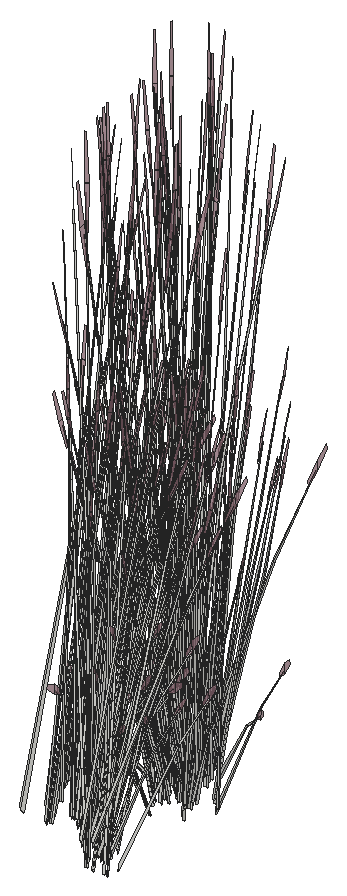
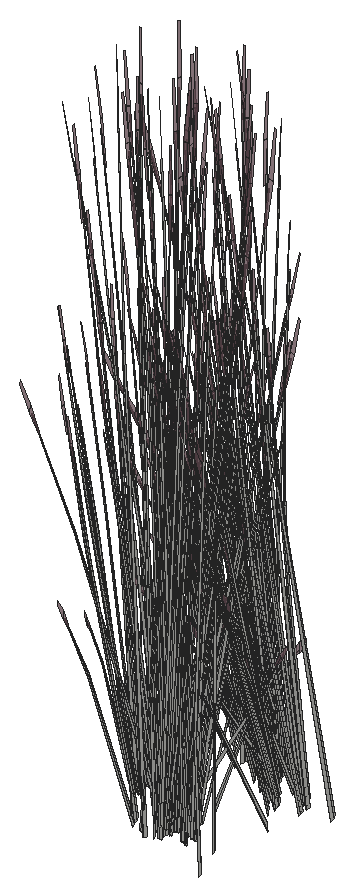
# SketchUp Ruby script. Lengths in inches.
U = 1.inch
M = Sketchup.active_model
def pt(a) = Geom::Point3d.new(a.map { |v| v * U })
def face(e, loops, mat)
  f = e.add_face(loops[0].map { |a| pt(a) })
  loops[1..].each { |l| e.add_face(l.map { |a| pt(a) }).erase! }
  f.material = f.back_material = mat if mat
  f
end
# faces: each face lists its corners as indices into pts; further lists are holes
def faces(e, pts, list, mat = nil) = list.each { |f| face(e, (f[0].is_a?(Array) ? f : [f]).map { |l| l.map { |i| pts[i] } }, mat) }
# xy, xz, yz: faces in a plane at the given z, y or x. An outline is a flat list of corners, or four numbers for a rectangle; further outlines are holes
def ring(l) = l.size == 4 ? [[l[0], l[1]], [l[2], l[1]], [l[2], l[3]], [l[0], l[3]]] : l.each_slice(2).to_a
def flat(e, list, mat, &to3) = list.each { |f| face(e, (f[0].is_a?(Array) ? f : [f]).map { |l| ring(l).map { |u, v| to3.(u, v) } }, mat) }
def xy(e, z, list, mat = nil) = flat(e, list, mat) { |x, y| [x, y, z] }
def xz(e, y, list, mat = nil) = flat(e, list, mat) { |x, z| [x, y, z] }
def yz(e, x, list, mat = nil) = flat(e, list, mat) { |y, z| [x, y, z] }
def lines(e, pts, list) = list.each { |a, b| e.add_line(pt(pts[a]), pt(pts[b])) }
# prism: a flat outline (further loops are holes) pulled along v
def prism(e, loops, v, mat = nil)
  f = face(e, loops, mat); d = Geom::Vector3d.new(v.map { |x| x * U })
  f.pushpull(f.normal.samedirection?(d) ? d.length : -d.length)
end
def box(e, o, s, mat = nil) = prism(e, [[o, [o[0] + s[0], o[1], o[2]], [o[0] + s[0], o[1] + s[1], o[2]], [o[0], o[1] + s[1], o[2]]]], [0, 0, s[2]], mat)
def at(x, y, z, deg = 0) = Geom::Transformation.translation(pt([x, y, z])) * Geom::Transformation.rotation(ORIGIN, Z_AXIS, deg.degrees)
def axes(o, x, y, z) = Geom::Transformation.new([*x, 0, *y, 0, *z, 0, *pt(o).to_a, 1])
def part(name) = M.definitions.add(name)
# library, detail: a bought-in or finely detailed component or shape, given as its bounding box
def library(name, o, s) = part(name).tap { |d| box(d.entities, o, s) }
def detail(e, o, s) = box(e.add_group.entities, o, s)
def put(e, d, t, mat = nil) = e.add_instance(d, t).tap { |i| i.material = mat if mat }
def group(e, t, mat = nil) = e.add_group.tap { |g| g.transformation = t; g.material = mat if mat }.entities
root = M.entities
M.materials.add("LightPink_Translucent").color = [144, 107, 117]
M.materials["LightPink_Translucent"].alpha = 0.75
c1 = part("blade")
p = [[2.15,0.21,22],[0,0.17,0],[0.09,0.45,0],[2.18,0.31,22],[2.29,0.31,22],[0.38,0.45,0],
  [2.48,0.24,33],[2.49,0.24,33],[2.48,0.22,33]]
faces(c1.entities,p,[[0,1,2,3],[4,5,2,3],[6,3,4,7],[8,0,3,6]])
c2 = part("seeds")
p = [[0.3,-0.1,1.38],[-0.01,-0.03,1.59],[-0.01,-0.03,0.03],[0.14,-0.07,-0.07],[0.29,-0.03,3],[0.15,0.01,3.11]]
faces(c2.entities,p,[[0,1,2,3],[1,0,4,5]],"LightPink_Translucent")
c3 = part("blade with seeds")
put(c3.entities,c1,at(0,0,0))
put(c3.entities,c2,axes([2.4,0.25,30.99],[1.5799,-0.05474,1.17369],[-0.12525,1.92788,0.29478],[-0.07173,-0.02425,1.56792]))
put(root,c3,axes([412.95,18.97,-7.78],[0.29098,0.34031,-0.32977],[-0.33226,0.32215,0.42575],[0.16881,0.04902,0.81462]))
put(root,c3,axes([413.09,18.02,-10.11],[-0.35699,0.33913,-0.28847],[-0.35699,-0.33913,0.28847],[0,0.10923,1.29413]))
put(root,c3,axes([411.55,18.05,-9.52],[0.05959,0.62022,-0.27094],[-0.62068,0.0375,-0.46562],[-0.1093,0.08261,1.4872]))
put(root,c3,axes([412.8,19.1,-7.6],[-0.02575,0.41332,0.05988],[-0.38885,-0.01133,0.47138],[0.14895,0.04325,0.71878]))
put(root,c3,axes([406.32,22.01,-7.6],[0.35109,0.22859,0.05988],[-0.2044,0.32553,0.47138],[0.11256,-0.10524,0.71878]))
put(root,c3,axes([411.78,17.8125,-9.94],[-0.24813,0.48978,-0.41661],[-0.51557,-0.23571,0.2005],[0,0.1129,1.33761]))
put(root,c3,axes([406.23,21.91,-7.59],[0.12683,0.50025,0.447],[-0.49754,0.08682,0.36857],[0.14663,-0.11765,0.92496]))
put(root,c3,axes([407.57,22.51,-7.61],[0.07097,-0.08279,1.62908],[-0.09083,-0.50786,-0.25764],[0.17806,-0.09629,0.13065]))
put(root,c3,axes([412.84,18.97,-7.59],[-0.37709,0.35815,0.447],[-0.32522,-0.38035,0.36857],[0.17692,0.06607,0.92496]))
put(root,c3,axes([407.98,19.35,-6.74],[0.45129,0.14509,-0.06041],[-0.13882,0.44656,-0.27392],[-0.07381,0.0678,0.90349]))
put(root,c3,axes([411.18,18.53,-10.08],[-0.34446,0.40855,-0.58063],[-0.42791,-0.37046,-0.15239],[-0.13803,0.10191,1.28164]))
put(root,c3,axes([411.64,19.38,-7.3],[-0.07899,-0.43781,0.32977],[0.45153,-0.11561,-0.42575],[0.12128,0.12546,0.81462]))
put(root,c3,axes([411.79,19.22,-9.83],[0.64025,0.17667,0.2864],[-0.16018,0.63149,-0.33981],[-0.10597,0.07904,1.53541]))
put(root,c3,axes([411.75,19.64,-10.12],[-0.47863,0.27177,-0.46235],[-0.28609,-0.48733,0],[-0.10901,0.0619,1.46668]))
put(root,c3,axes([413.34,18.03,-10.12],[0,0.54355,-0.46235],[-0.57217,0,0],[0,0.1238,1.46668]))
put(root,c3,axes([411.91,18.09,-8.39],[-0.18996,-0.09365,1.59586],[0.39312,-0.39287,0.12904],[0.24502,0.17723,0.68222]))
put(root,c3,axes([411.94,16.86,-7.83],[-0.44191,-0.28242,1.28769],[0.46662,-0.43971,0.5556],[0.14258,0.26499,1.24467]))
put(root,c3,axes([412.61,19.16,-9.42],[-0.28795,-0.15629,1.06958],[0.37181,-0.1588,0.78586],[0.10029,0.13452,0.23558]))
put(root,c3,axes([406.17,23.29,-7.3125],[-0.25732,-0.49218,-0.11324],[0.45669,-0.24187,-0.62851],[0.19245,-0.06494,0.95501]))
put(root,c3,axes([406.15,22.86,-7.64],[0.13855,-0.49442,-0.47583],[0.47502,0.16947,-0.36857],[0.19125,-0.04534,0.91046]))
put(root,c3,axes([411.6,19.61,-7.3125],[0.30474,-0.46525,-0.11324],[0.44133,0.26804,-0.62851],[0.15341,0.13145,0.95501]))
put(root,c3,axes([405.4,20.85,-9.79],[0.31974,-0.54466,0],[0.53494,0.30375,-0.48057],[0.12184,0.06918,1.52448]))
put(root,c3,axes([406.65,23,-10.15],[-0.32938,0.06523,1.31842],[-0.05243,-0.51922,0.07547],[0.2307,-0.07859,0.75023]))
put(root,c3,axes([407.25,22.54,-9.89],[-0.31706,-0.34757,-0.06041],[0.34725,-0.31847,-0.27392],[0.09839,-0.02242,0.90349]))
put(root,c3,axes([409.59,18.98,-7.3],[0.34603,-0.28618,0.32977],[0.32756,0.32677,-0.42575],[-0.04984,0.16603,0.81462]))
put(root,c3,axes([412.18,19.56,-9.79],[0.31974,0.54466,0],[-0.53494,0.30375,-0.48057],[-0.12184,0.06918,1.52448]))
put(root,c3,axes([411.2,19.99,-7.62],[0.00151,-0.06581,1.65179],[0.43826,-0.29033,-0.15608],[0.15223,0.10363,0.29231]))
put(root,c3,axes([412.6875,19.74,-10.61],[0.03726,-0.07847,1.6421],[0.46909,-0.23111,-0.25086],[0.14221,0.11962,0.2797]))
put(root,c3,axes([411.91,17.4,-9.35],[-0.01397,-0.51177,1.31553],[0.63227,0.13266,0.557],[-0.14954,0.28003,1.24175]))
put(root,c3,axes([412.07,17.96,-10.05],[0.18752,0.49766,-0.6445],[-0.54017,0.17923,-0.16915],[0.02073,0.16852,1.42262]))
put(root,c3,axes([409.27,19.24,-7.6],[-0.42027,-0.02533,0.05988],[0.01152,-0.38243,0.47138],[-0.04398,0.14649,0.71878]))
put(root,c3,axes([406.06,23.04,-7.36],[0.44939,-0.24006,-0.66157],[0.25044,0.49415,0.07984],[0.21713,-0.05613,0.93586]))
put(root,c3,axes([409.41,19.27,-7.59],[-0.36417,-0.37086,0.447],[0.38674,-0.31985,0.36857],[-0.06718,0.174,0.92496]))
put(root,c3,axes([411.96,19.375,-7.64],[0.50465,-0.12921,-0.47583],[0.08828,0.48932,-0.36857],[0.13555,0.14022,0.91046]))
put(root,c3,axes([410.56,19.45,-7.3],[0.15418,-0.41799,0.32977],[0.44981,0.12192,-0.42575],[0.04124,0.16829,0.81462]))
put(root,c3,axes([405.99,23.14,-7.3],[-0.42502,-0.15163,0.32977],[0.12396,-0.44238,-0.42575],[0.17112,-0.04056,0.81462]))
put(root,c3,axes([412.65,19.87,-9.52],[-0.32795,-0.01705,0.97832],[0.21658,-0.36206,0.54015],[0.12956,0.12863,0.76741]))
put(root,c3,axes([403.08,21.82,-10.52],[-0.50338,0.21762,1.20058],[-0.16022,-0.62439,0.4665],[0.30911,0.01039,1.36553]))
put(root,c3,axes([411.71,19.78,-7.6],[-0.23243,0.34529,0.05988],[-0.331,-0.20103,0.47138],[0.10701,0.1107,0.71878]))
put(root,c3,axes([411.16,20.94,-6.74],[0.35341,-0.31182,-0.06041],[0.32382,0.34152,-0.27392],[0.0228,0.09677,0.90349]))
put(root,c3,axes([407.01,22.66,-10.61],[-0.02673,-0.08252,1.6421],[0.18538,-0.48271,-0.25086],[0.187,-0.00694,0.2797]))
put(root,c3,axes([411.81,19.68,-7.59],[-0.50866,0.12474,0.447],[-0.08828,-0.48932,0.36857],[0.11963,0.14421,0.92496]))
put(root,c3,axes([411.58,18.99,-9.59],[0.00902,-0.18018,1.33163],[0.43127,-0.20126,-0.28638],[0.13313,0.21566,0.56934]))
put(root,c3,axes([404.39,22.14,-9.52],[0.51635,-0.36087,-0.27094],[0.34336,0.5099,-0.46562],[0.1274,0.05178,1.4872]))
put(root,c3,axes([406.4375,23.09,-7.78],[0.42502,0.15163,-0.32977],[-0.12396,0.44238,0.42575],[0.17112,-0.04056,0.81462]))
put(root,c3,axes([410.42,19.83,-7.6],[-0.37684,0.18473,0.05988],[-0.18445,-0.33686,0.47138],[0.03639,0.14849,0.71878]))
put(root,c3,axes([409.41,19.38,-7.78],[-0.34603,0.28618,-0.32977],[-0.32756,-0.32677,0.42575],[-0.04984,0.16603,0.81462]))
put(root,c3,axes([409.37,19.06,-6.97],[0.56206,0.02693,-0.12569],[-0.01536,0.50991,-0.69765],[-0.03904,0.19638,1.06006]))
put(root,c3,axes([410.41,19.625,-7.3125],[0.50045,-0.25306,-0.11324],[0.24593,0.44915,-0.62851],[0.06603,0.18927,0.95501]))
put(root,c3,axes([405.6875,21.18,-10.12],[0.47863,0.27177,-0.46235],[-0.28609,0.48733,0],[0.10901,0.0619,1.46668]))
put(root,c3,axes([410.55,19.79,-7.28],[-0.50393,-0.1421,0.49617],[0.17232,-0.46717,0.40911],[0.03028,0.18372,1.0267]))
put(root,c3,axes([409.63,20.5,-9.42],[-0.01324,-0.32319,1.06958],[0.33072,0.23052,0.78586],[-0.06504,0.15405,0.23558]))
put(root,c3,axes([410.5,19.72,-10.61],[0.08277,-0.02958,1.6421],[0.49786,0.16279,-0.25086],[0.01456,0.18348,0.2797]))
put(root,c3,axes([405.28,22.54,-8.39],[-0.21212,0.01231,1.59586],[0.14072,-0.53355,0.12904],[0.3023,0.033,0.68222]))
put(root,c3,axes([405.55,21.38,-10.11],[0.12013,0.47362,-0.28847],[-0.47712,0.13449,0.28847],[0.09619,0.05462,1.29413]))
put(root,c3,axes([406.375,23.28,-7.6],[0.18783,0.37061,0.05988],[-0.34252,0.1814,0.47138],[0.15099,-0.03579,0.71878]))
put(root,c3,axes([409.75,19.25,-7.34],[0.3661,0.36521,-0.52818],[-0.38674,0.31985,-0.40911],[-0.0557,0.18556,1.01061]))
put(root,c3,axes([406.34,23.14,-7.59],[-0.14449,0.4956,0.447],[-0.47502,-0.16947,0.36857],[0.1868,-0.02978,0.92496]))
put(root,c3,axes([409.35,19.8,-9.37],[0.46459,-0.09625,0.0606],[0.10681,0.38778,-0.80367],[-0.02945,0.1963,0.72038]))
put(root,c3,axes([410.84,19.6,-7.64],[0.50273,0.13626,-0.47583],[-0.17232,0.46717,-0.36857],[0.0461,0.18809,0.91046]))
put(root,c3,axes([411.12,18.64,-8.39],[-0.1169,-0.17452,1.59586],[0.54019,-0.14692,0.12904],[0.12209,0.27397,0.68222]))
put(root,c3,axes([409.73,26.76,-7.61],[-0.07822,-0.07621,1.62908],[-0.52201,0.04832,-0.25764],[-0.08331,-0.18228,0.13065]))
put(root,c3,axes([410.94,27.67,-9.59],[-0.14537,0.11002,1.33163],[-0.43536,-0.19256,-0.28638],[0.0807,-0.23948,0.56934]))
put(root,c3,axes([410.28,28.05,-7.36],[-0.24409,-0.44196,-0.66157],[0.50245,-0.2463,0.07984],[-0.05708,-0.21354,0.93586]))
put(root,c3,axes([410.61,19.89,-7.78],[-0.15418,0.41799,-0.32977],[-0.44981,-0.12192,0.42575],[0.04124,0.16829,0.81462]))
put(root,c3,axes([409.64,19.08,-7.03],[-0.01331,0.50278,-0.73435],[-0.56035,-0.03377,0.08862],[-0.05914,0.213,1.03881]))
put(root,c3,axes([404.99,22.22,-10.08],[0.53199,0.08911,-0.58063],[-0.11226,0.54969,-0.15239],[0.15876,0.06661,1.28164]))
put(root,c3,axes([408.17,20.4,-7.62],[0.05802,-0.03282,1.65179],[0.47954,0.21828,-0.15608],[-0.01127,0.18175,0.29231]))
put(root,c3,axes([407.34,23.18,-9.42],[-0.31598,0.08973,1.06958],[0.14873,-0.37085,0.78586],[0.16763,0.02538,0.23558]))
put(root,c3,axes([409.86,27.07,-10.61],[-0.08578,0.01958,1.6421],[-0.47437,-0.22044,-0.25086],[0.00796,-0.18387,0.2797]))
put(root,c3,axes([410.17,18.73,-8.39],[-0.01252,-0.20862,1.59586],[0.54251,0.1384,0.12904],[-0.03356,0.2973,0.68222]))
put(root,c3,axes([411.29,28.48,-7.36],[0.01331,-0.50278,-0.66157],[0.56035,0.03377,0.07984],[0.05914,-0.213,0.93586]))
put(root,c3,axes([407.19,24.75,-7.62],[-0.04624,-0.04758,1.65179],[0.10116,-0.51007,-0.15608],[0.18215,-0.03259,0.29231]))
put(root,c3,axes([412.08,27.7,-7.61],[-0.00494,-0.10818,1.62908],[-0.41695,-0.31265,-0.25764],[0.06446,-0.18952,0.13065]))
put(root,c3,axes([410.32,27.67,-7.78],[0.15418,-0.41799,-0.32977],[0.44981,0.12192,0.42575],[-0.04124,-0.16829,0.81462]))
put(root,c3,axes([410.66,28.23,-8.39],[-0.09522,0.18683,1.59586],[-0.39947,-0.38663,0.12904],[0.18021,-0.24097,0.68222]))
put(root,c3,axes([411.96,27.31,-7.62],[-0.05194,0.04152,1.65179],[-0.50886,-0.14007,-0.15608],[-0.01842,-0.18118,0.29231]))
put(root,c3,axes([410.65,19.51,-7.36],[0.24409,0.44196,-0.66157],[-0.50245,0.2463,0.07984],[0.05708,0.21354,0.93586]))
put(root,c3,axes([406.79,24.32,-8.34],[-0.09788,-0.45691,-0.03251],[0.46264,-0.10504,-0.14742],[0.09661,0.02897,0.48626]))
put(root,c3,axes([409.24,20.21,-9.59],[0.16138,-0.08575,1.33163],[0.39845,0.25854,-0.28638],[-0.1186,0.22371,0.56934]))
put(root,c3,axes([405.59,24.31,-7.3125],[0.02738,-0.55277,-0.11324],[0.51847,0.01511,-0.62851],[0.19968,0.0384,0.95501]))
put(root,c3,axes([410.29,20.63,-7.61],[0.06483,0.08753,1.62908],[0.52315,0.03439,-0.25764],[0.05261,0.19303,0.13065]))
put(root,c3,axes([410.09,27.96,-7.64],[-0.50273,-0.13626,-0.47583],[0.17232,-0.46717,-0.36857],[-0.0461,-0.18809,0.91046]))
put(root,c3,axes([410.41,26.79,-9.42],[0.06561,0.31695,1.06958],[-0.36394,-0.17555,0.78586],[0.03916,-0.16229,0.23558]))
put(root,c3,axes([411.18,28.31,-7.64],[-0.3661,-0.36521,-0.47583],[0.38674,-0.31985,-0.36857],[0.0557,-0.18556,0.91046]))
put(root,c3,axes([405.51,24.09,-7.3],[-0.29098,-0.34031,0.32977],[0.33226,-0.32215,-0.42575],[0.16881,0.04902,0.81462]))
put(root,c3,axes([406.75,23.77,-9.59],[-0.12317,-0.13368,1.33163],[0.16025,-0.44223,-0.28638],[0.24919,0.05991,0.56934]))
put(root,c3,axes([409.09,27.67,-7.26],[0.56969,-0.13971,0.50064],[0.09887,0.54803,0.4128],[-0.13398,-0.16152,1.03595]))
put(root,c3,axes([410.38,27.77,-7.59],[0.50393,0.1421,0.447],[-0.17232,0.46717,0.36857],[-0.03028,-0.18372,0.92496]))
put(root,c3,axes([410.52,27.9375,-7.3125],[-0.50045,0.25306,-0.11324],[-0.24593,-0.44915,-0.62851],[-0.06603,-0.18927,0.95501]))
put(root,c3,axes([411.5625,28.51,-7.3125],[-0.56206,-0.02693,-0.11324],[0.01536,-0.50991,-0.62851],[0.03904,-0.19638,0.95501]))
put(root,c3,axes([411.53,28.18,-7.78],[0.34603,-0.28618,-0.32977],[0.32756,0.32677,0.42575],[0.04984,-0.16603,0.81462]))
put(root,c3,axes([409.45,19.79,-8.87],[0.01124,-0.2806,1.43727],[0.50537,0.14821,0.19862],[-0.04379,0.29905,0.67868]))
put(root,c3,axes([408.53,27.17,-9.42],[0.26677,0.18918,1.06958],[-0.38851,0.11372,0.78586],[-0.08313,-0.14539,0.23558]))
put(root,c3,axes([410.51,27.74,-7.6],[0.37684,-0.18473,0.05988],[0.18445,0.33686,0.47138],[-0.03639,-0.14849,0.71878]))
put(root,c3,axes([406.04,23.98,-7.61],[0.10971,-0.00919,1.62908],[0.30091,-0.42228,-0.25764],[0.19514,0.05574,0.13065]))
put(root,c3,axes([405.62,24.04,-7.36],[0.51122,0.01309,-0.66157],[-0.03434,0.5511,0.07984],[0.21658,0.05816,0.93586]))
put(root,c3,axes([409.22,27.79,-7.6],[0.23243,-0.34529,0.05988],[0.331,0.20103,0.47138],[-0.10701,-0.1107,0.71878]))
put(root,c3,axes([409.15,29.71,-10.05],[-0.21003,-0.55738,-0.65031],[0.60499,-0.20074,-0.17068],[-0.02321,-0.18874,1.43544]))
put(root,c3,axes([411.96,28.01,-10.61],[-0.07655,-0.04282,1.6421],[-0.19662,-0.47839,-0.25086],[0.13264,-0.12982,0.2797]))
put(root,c3,axes([406.45,22.92,-9.79],[0.63949,0,0],[0,0.60749,-0.48057],[0,0.13836,1.52448]))
put(root,c3,axes([410.375,28.11,-7.3],[-0.15418,0.41799,0.32977],[-0.44981,-0.12192,-0.42575],[-0.04124,-0.16829,0.81462]))
put(root,c3,axes([405.92,24.27,-7.78],[0.29098,0.34031,-0.32977],[-0.33226,0.32215,0.42575],[0.16881,0.04902,0.81462]))
put(root,c3,axes([411.52,28.29,-7.59],[0.36417,0.37086,0.447],[-0.38674,0.31985,0.36857],[0.06718,-0.174,0.92496]))
put(root,c3,axes([405.78,24.4,-7.6],[-0.02575,0.41332,0.05988],[-0.38885,-0.01133,0.47138],[0.14895,0.04325,0.71878]))
put(root,c3,axes([411.66,28.33,-7.6],[0.42027,0.02533,0.05988],[-0.01152,0.38243,0.47138],[0.04398,-0.14649,0.71878]))
put(root,c3,axes([405.8125,24.27,-7.59],[-0.37709,0.35815,0.447],[-0.32522,-0.38035,0.36857],[0.17692,0.06607,0.92496]))
put(root,c3,axes([411.34,28.59,-7.3],[-0.34603,0.28618,0.32977],[-0.32756,-0.32677,-0.42575],[0.04984,-0.16603,0.81462]))
put(root,c3,axes([411.95,29.36,-7.36],[0.26714,-0.42887,-0.66157],[0.46811,0.30479,0.07984],[0.1595,-0.15539,0.93586]))
put(root,c3,axes([409.07,28.11,-9.79],[-0.31974,-0.54466,0],[0.53494,-0.30375,-0.48057],[0.12184,-0.06918,1.52448]))
put(root,c3,axes([411.94,29.16,-7.64],[-0.13138,-0.49631,-0.47583],[0.49754,-0.08682,-0.36857],[0.14258,-0.13331,0.91046]))
put(root,c3,axes([409.77,27.45,-10.02],[-0.35341,0.31182,-0.03625],[-0.32382,-0.34152,-0.16435],[-0.0228,-0.09677,0.54209]))
put(root,c3,axes([412.18,29.51,-7.3125],[-0.47307,-0.29971,-0.11324],[0.27254,-0.43404,-0.62851],[0.13365,-0.15087,0.95501]))
put(root,c3,axes([404.88,23.4,-8.39],[-0.18996,-0.09365,1.59586],[0.39312,-0.39287,0.12904],[0.24502,0.17723,0.68222]))
put(root,c3,axes([407.91,29.63,-10.12],[0,-0.54355,-0.46235],[0.57217,0,0],[0,-0.1238,1.46668]))
put(root,c3,axes([409.5,28.02,-10.12],[0.47863,-0.27177,-0.46235],[0.28609,0.48733,0],[0.10901,-0.0619,1.46668]))
put(root,c3,axes([412.34,28.96,-9.59],[-0.1827,-0.0161,1.33163],[-0.18717,-0.43188,-0.28638],[0.22444,-0.12218,0.56934]))
put(root,c3,axes([413.34,29.38,-7.62],[-0.0668,-0.00413,1.65179],[-0.27738,-0.44233,-0.15608],[0.11139,-0.14544,0.29231]))
put(root,c3,axes([404.57,24.91,-7.3125],[0.30474,-0.46525,-0.11324],[0.44133,0.26804,-0.62851],[0.15341,0.13145,0.95501]))
put(root,c3,axes([410.07,29.14,-10.08],[0.34446,-0.40855,-0.58063],[0.42791,0.37046,-0.15239],[0.13803,-0.10191,1.28164]))
put(root,c3,axes([412.55,28.17,-9.42],[-0.17034,0.27669,1.06958],[-0.14642,-0.37174,0.78586],[0.14069,-0.09315,0.23558]))
put(root,c3,axes([412.31,29.21,-7.78],[0.44516,-0.07768,-0.32977],[0.11755,0.44407,0.42575],[0.12757,-0.11927,0.81462]))
put(root,c3,axes([405.66,25.04,-10.61],[0.03726,-0.07847,1.6421],[0.46909,-0.23111,-0.25086],[0.14221,0.11962,0.2797]))
put(root,c3,axes([404.93,24.68,-7.64],[0.50465,-0.12921,-0.47583],[0.08828,0.48932,-0.36857],[0.13555,0.14022,0.91046]))
put(root,c3,axes([409.47,29.85,-9.94],[0.24813,-0.48978,-0.41661],[0.51557,0.23571,0.2005],[0,-0.1129,1.33761]))
put(root,c3,axes([409.69,29.61,-9.52],[-0.05959,-0.62022,-0.27094],[0.62068,-0.0375,-0.46562],[0.1093,-0.08261,1.4872]))
put(root,c3,axes([408.16,29.64,-10.11],[0.35699,-0.33913,-0.28847],[0.35699,0.33913,0.28847],[0,-0.10923,1.29413]))
put(root,c3,axes([411.95,29.47,-7.3],[-0.44516,0.07768,0.32977],[-0.11755,-0.44407,-0.42575],[0.12757,-0.11927,0.81462]))
put(root,c3,axes([409.41,30.26,-9.52],[-0.57594,-0.25935,-0.27094],[0.27732,-0.5474,-0.46562],[-0.0181,-0.1344,1.4872]))
put(root,c3,axes([405.63,25.18,-9.52],[-0.32795,-0.01705,0.97832],[0.21658,-0.36206,0.54015],[0.12956,0.12863,0.76741]))
put(root,c3,axes([409.61,28.24,-10.11],[0.47712,0.13449,-0.28847],[-0.12013,0.47362,0.28847],[0.09619,-0.05462,1.29413]))
put(root,c3,axes([412.35,29.4,-7.6],[0.35109,0.22859,0.05988],[-0.2044,0.32553,0.47138],[0.11256,-0.10524,0.71878]))
put(root,c3,axes([412.25,29.3,-7.59],[0.12683,0.50025,0.447],[-0.49754,0.08682,0.36857],[0.14663,-0.11765,0.92496]))
put(root,c3,axes([413.59,29.91,-7.61],[0.07097,-0.08279,1.62908],[-0.09083,-0.50786,-0.25764],[0.17806,-0.09629,0.13065]))
put(root,c3,axes([409.78,30.1,-9.73],[0.57623,0.26344,0.22409],[-0.27732,0.5474,0.46562],[0,-0.12618,1.49497]))
put(root,c3,axes([409.55,30.84,-9.73],[0.13555,-0.64407,-0.21817],[0.64269,0.11227,0.47743],[-0.1123,-0.08895,1.45677]))
put(root,c3,axes([409.59,29.73,-9.47],[-0.55535,0.03355,0.41661],[-0.05022,-0.55698,-0.2005],[0.09942,-0.05645,1.33761]))
put(root,c3,axes([404.26,32.82,-8.39],[-0.09522,0.18683,1.59586],[-0.39947,-0.38663,0.12904],[0.18021,-0.24097,0.68222]))
put(root,c3,axes([408.16,30.14,-9.69],[0,0.54355,0.46235],[-0.57217,0,0],[0,-0.1238,1.46668]))
put(root,c3,axes([412.2,30.68,-7.3125],[-0.25732,-0.49218,-0.11324],[0.45669,-0.24187,-0.62851],[0.19245,-0.06494,0.95501]))
put(root,c3,axes([412.17,30.26,-7.64],[0.13855,-0.49442,-0.47583],[0.47502,0.16947,-0.36857],[0.19125,-0.04534,0.91046]))
put(root,c3,axes([411.42,28.24,-9.79],[0.31974,-0.54466,0],[0.53494,0.30375,-0.48057],[0.12184,0.06918,1.52448]))
put(root,c3,axes([409.51,30.57,-9.94],[-0.30722,-0.45622,-0.41661],[0.46535,-0.32126,0.2005],[-0.09942,-0.05645,1.33761]))
put(root,c3,axes([409.57,29.93,-9.8],[0.22235,0.6078,0.42607],[-0.63531,0.21135,0.16719],[0.00776,-0.11168,1.47927]))
put(root,c3,axes([412.68,30.4,-10.15],[-0.32938,0.06523,1.31842],[-0.05243,-0.51922,0.07547],[0.2307,-0.07859,0.75023]))
put(root,c3,axes([413.28,29.9375,-9.89],[-0.31706,-0.34757,-0.06041],[0.34725,-0.31847,-0.27392],[0.09839,-0.02242,0.90349]))
put(root,c3,axes([409.46,30.41,-9.47],[-0.24813,0.48978,0.41661],[-0.51557,-0.23571,-0.2005],[0,-0.1129,1.33761]))
put(root,c3,axes([410.37,29.98,-9.95],[0,-0.62892,0],[0.63949,0,0],[0,0,1.6711]))
put(root,c3,axes([411.15,28.53,-9.69],[-0.47863,-0.27177,0.46235],[0.28609,-0.48733,0],[0.10901,0.0619,1.46668]))
put(root,c3,axes([412.08,30.4375,-7.36],[0.44939,-0.24006,-0.66157],[0.25044,0.49415,0.07984],[0.21713,-0.05613,0.93586]))
put(root,c3,axes([410.07,29.59,-9.8],[-0.42403,0.49328,0.42607],[-0.50377,-0.43543,0.16719],[0.10223,-0.04923,1.47927]))
put(root,c3,axes([410.53,30.47,-9.86],[-0.47569,-0.46784,-0.05709],[0.47598,-0.46812,0],[-0.01661,-0.01634,1.63492]))
put(root,c3,axes([409.33,28.77,-9.7],[-0.14774,0.54019,0.16428],[-0.54062,-0.15287,0.32672],[0.09339,-0.00263,1.49371]))
put(root,c3,axes([412.02,30.53,-7.3],[-0.42502,-0.15163,0.32977],[0.12396,-0.44238,-0.42575],[0.17112,-0.04056,0.81462]))
put(root,c3,axes([409.11,29.21,-10.52],[-0.50338,0.21762,1.20058],[-0.16022,-0.62439,0.4665],[0.30911,0.01039,1.36553]))
put(root,c3,axes([410.46,29.375,-9.5625],[0.09866,-0.48509,0.13483],[0.48202,0.0842,-0.38503],[0.08772,0.04981,1.18024]))
put(root,c3,axes([409.625,30.53,-9.8],[0.64638,0.11452,0.42607],[-0.13155,0.64678,0.16719],[-0.09446,-0.06245,1.47927]))
put(root,c3,axes([413.04,30.06,-10.61],[-0.02673,-0.08252,1.6421],[0.18538,-0.48271,-0.25086],[0.187,-0.00694,0.2797]))
put(root,c3,axes([410.25,29.5,-9.47],[-0.30722,-0.45622,0.41661],[0.46535,-0.32126,-0.2005],[0.09942,0.05645,1.33761]))
put(root,c3,axes([409.28,31.56,-9.7],[0.54955,-0.14427,0.16428],[0.1357,0.53689,0.32672],[-0.04901,-0.07823,1.49371]))
put(root,c3,axes([410.41,29.53,-9.52],[0.51635,-0.36087,-0.27094],[0.34336,0.5099,-0.46562],[0.1274,0.05178,1.4872]))
put(root,c3,axes([412.46,30.48,-7.78],[0.42502,0.15163,-0.32977],[-0.12396,0.44238,0.42575],[0.17112,-0.04056,0.81462]))
put(root,c3,axes([405.56,32.6,-10.61],[-0.07655,-0.04282,1.6421],[-0.19662,-0.47839,-0.25086],[0.13264,-0.12982,0.2797]))
put(root,c3,axes([411.71,28.57,-10.12],[0.47863,0.27177,-0.46235],[-0.28609,0.48733,0],[0.10901,0.0619,1.46668]))
put(root,c3,axes([410.8,30.12,-9.95],[0.57217,0,0],[0,0.56272,0],[0,0,1.66132]))
put(root,c3,axes([410.97,28.8,-9.7],[-0.54955,0.14427,0.16428],[-0.1357,-0.53689,0.32672],[0.04901,0.07823,1.49371]))
put(root,c3,axes([411.31,29.94,-8.39],[-0.21212,0.01231,1.59586],[0.14072,-0.53355,0.12904],[0.3023,0.033,0.68222]))
put(root,c3,axes([411.58,28.78,-10.11],[0.12013,0.47362,-0.28847],[-0.47712,0.13449,0.28847],[0.09619,0.05462,1.29413]))
put(root,c3,axes([405.55,33.95,-7.36],[0.26714,-0.42887,-0.66157],[0.46811,0.30479,0.07984],[0.1595,-0.15539,0.93586]))
put(root,c3,axes([412.4,30.67,-7.6],[0.18783,0.37061,0.05988],[-0.34252,0.1814,0.47138],[0.15099,-0.03579,0.71878]))
put(root,c3,axes([405.54,33.75,-7.64],[-0.13138,-0.49631,-0.47583],[0.49754,-0.08682,-0.36857],[0.14258,-0.13331,0.91046]))
put(root,c3,axes([410.62,29.84,-9.78],[-0.64638,-0.11452,0.45814],[0.13155,-0.64678,0.17978],[0.09446,0.06245,1.59061]))
put(root,c3,axes([412.37,30.54,-7.59],[-0.14449,0.4956,0.447],[-0.47502,-0.16947,0.36857],[0.1868,-0.02978,0.92496]))
put(root,c3,axes([410.1,31.43,-9.95],[-0.16686,-0.46861,0],[0.47648,-0.16411,0],[0,0,1.4375]))
put(root,c3,axes([409.79,30.99,-9.5625],[-0.09866,0.48509,0.13483],[-0.48202,-0.0842,-0.38503],[-0.08772,-0.04981,1.18024]))
put(root,c3,axes([410.73,31.37,-9.97],[0.53691,-0.18442,-0.17877],[0.18866,0.53125,0.00007],[0.05927,-0.02038,1.61933]))
put(root,c3,axes([405.78,34.1,-7.3125],[-0.47307,-0.29971,-0.11324],[0.27254,-0.43404,-0.62851],[0.13365,-0.15087,0.95501]))
put(root,c3,axes([410.91,31.59,-9.7],[0.14774,-0.54019,0.16428],[0.54062,0.15287,0.32672],[-0.09339,0.00263,1.49371]))
put(root,c3,axes([410.79,30.36,-9.9375],[0.35699,0.35109,0],[-0.35699,0.35109,0],[0,0,1.57621]))
